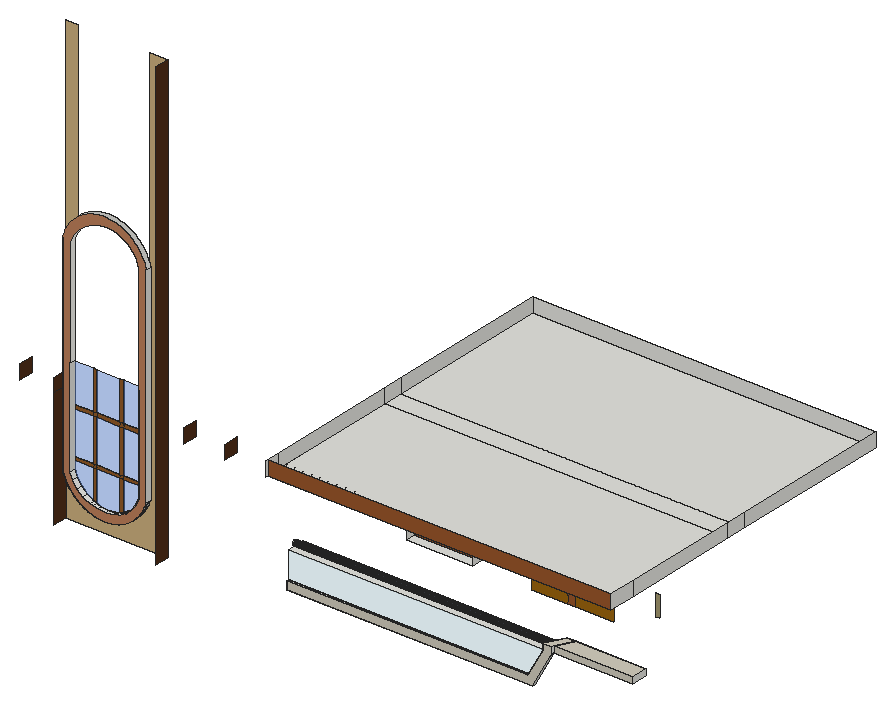
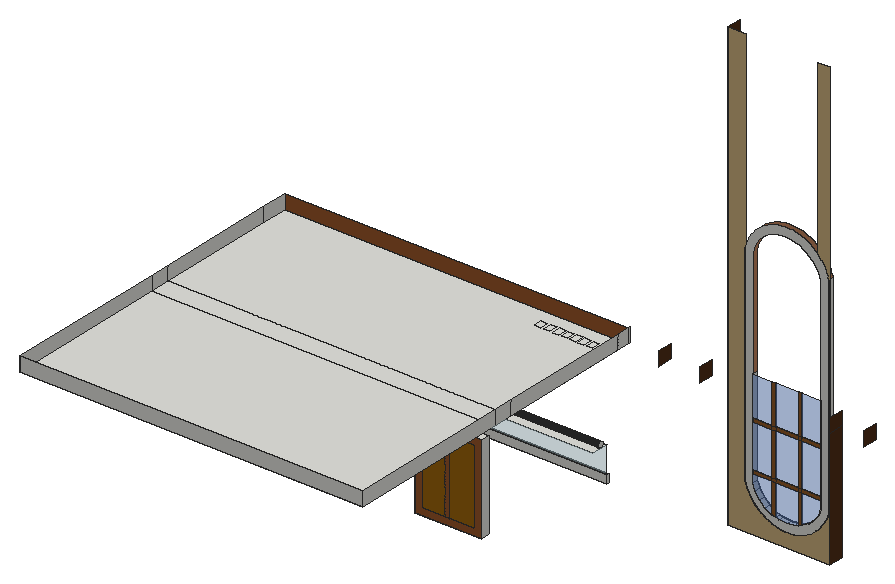
# SketchUp Ruby script. Lengths in inches.
U = 1.inch
M = Sketchup.active_model
def pt(a) = Geom::Point3d.new(a.map { |v| v * U })
def face(e, loops, mat)
  f = e.add_face(loops[0].map { |a| pt(a) })
  loops[1..].each { |l| e.add_face(l.map { |a| pt(a) }).erase! }
  f.material = f.back_material = mat if mat
  f
end
# faces: each face lists its corners as indices into pts; further lists are holes
def faces(e, pts, list, mat = nil) = list.each { |f| face(e, (f[0].is_a?(Array) ? f : [f]).map { |l| l.map { |i| pts[i] } }, mat) }
# xy, xz, yz: faces in a plane at the given z, y or x. An outline is a flat list of corners, or four numbers for a rectangle; further outlines are holes
def ring(l) = l.size == 4 ? [[l[0], l[1]], [l[2], l[1]], [l[2], l[3]], [l[0], l[3]]] : l.each_slice(2).to_a
def flat(e, list, mat, &to3) = list.each { |f| face(e, (f[0].is_a?(Array) ? f : [f]).map { |l| ring(l).map { |u, v| to3.(u, v) } }, mat) }
def xy(e, z, list, mat = nil) = flat(e, list, mat) { |x, y| [x, y, z] }
def xz(e, y, list, mat = nil) = flat(e, list, mat) { |x, z| [x, y, z] }
def yz(e, x, list, mat = nil) = flat(e, list, mat) { |y, z| [x, y, z] }
def lines(e, pts, list) = list.each { |a, b| e.add_line(pt(pts[a]), pt(pts[b])) }
# prism: a flat outline (further loops are holes) pulled along v
def prism(e, loops, v, mat = nil)
  f = face(e, loops, mat); d = Geom::Vector3d.new(v.map { |x| x * U })
  f.pushpull(f.normal.samedirection?(d) ? d.length : -d.length)
end
def box(e, o, s, mat = nil) = prism(e, [[o, [o[0] + s[0], o[1], o[2]], [o[0] + s[0], o[1] + s[1], o[2]], [o[0], o[1] + s[1], o[2]]]], [0, 0, s[2]], mat)
def at(x, y, z, deg = 0) = Geom::Transformation.translation(pt([x, y, z])) * Geom::Transformation.rotation(ORIGIN, Z_AXIS, deg.degrees)
def axes(o, x, y, z) = Geom::Transformation.new([*x, 0, *y, 0, *z, 0, *pt(o).to_a, 1])
def part(name) = M.definitions.add(name)
# library, detail: a bought-in or finely detailed component or shape, given as its bounding box
def library(name, o, s) = part(name).tap { |d| box(d.entities, o, s) }
def detail(e, o, s) = box(e.add_group.entities, o, s)
def put(e, d, t, mat = nil) = e.add_instance(d, t).tap { |i| i.material = mat if mat }
def group(e, t, mat = nil) = e.add_group.tap { |g| g.transformation = t; g.material = mat if mat }.entities
root = M.entities
M.materials.add("[Blinds Wood Light]").color = [155, 100, 14]
M.materials.add("[Formica Graystone]").color = [209, 204, 189]
M.materials.add("[Formica Laminate Dark]").color = [50, 53, 60]
M.materials.add("[Translucent Glass Blue]").color = [100, 149, 237]
M.materials["[Translucent Glass Blue]"].alpha = 0.5
M.materials.add("[Translucent Glass Safety]").color = [204, 235, 244]
M.materials["[Translucent Glass Safety]"].alpha = 0.5
M.materials.add("[Wood Board Cork]").color = [215, 201, 115]
M.materials.add("[Wood Cherry Original]").color = [152, 86, 42]
M.materials.add("[Wood Floor Light]").color = [204, 176, 127]
M.materials.add("[Wood Floor Parquet]").color = [145, 89, 39]
M.materials.add("[Wood Lumber ButtJoined]").color = [164, 152, 112]
M.materials.add("[Wood Veneer 01]").color = [79, 46, 24]
M.materials.add("[Wood Veneer 02]").color = [190, 128, 91]
xy(root,246.23,[[380.95,348.07,452.45,357.95]])
xy(root,246.97,[[356.6875,216.87,621.625,219.56]])
xy(root,255.23,[[356.6875,216.87,615.875,219.56]])
xy(root,284.4375,[[356.6875,219.56,632.125,219.56,641.9,237.64,356.6875,237.64],[632.125,219.56,641.9,237.64,651.75,237.64,641.9,219.56],[641.9,219.56,651.75,237.64,727.17,237.64,727.17,219.56]])
xy(root,291.5,[[632.125,216.87,641.9,216.87,641.9,219.56,651.75,237.64,641.9,237.64,632.125,219.56],[641.9,219.56,727.17,219.56,727.17,237.64,651.75,237.64]],"[Formica Graystone]")
xy(root,341.42,[[380.95,348.07,452.45,357.95]])
xy(root,369,[[356.6875,190.11,727.17,348.07],[358.51,205,364.9375,214.21],[367.14,205,373.5625,214.21],[376.01,205,382.4375,214.21],[385.08,205,391.5,214.21],
  [393.95,205,400.375,214.21],[403.08,205,409.5,214.21],[412.39,205,418.8125,214.21],[422.26,205,428.6875,214.21],[432.2,205,438.625,214.21],
  [356.6875,348.07,727.17,370.07],[356.6875,370.07,727.17,548.03]])
xz(root,190.11,[[356.6875,369,727.17,384.375]],"[Wood Cherry Original]")
xz(root,197.92,[[[174.5,257.11,176.5,257.16,178.5,257.29,180.5,257.5,182.48,257.8,184.45,258.18,186.4,258.65,188.33,259.2,190.24,259.83,192.11,260.54,193.96,261.33,195.76,262.2,197.53,263.15,199.26,264.17,200.94,265.26,202.58,266.43,204.16,267.66,205.6875,268.96,207.16,270.32,208.57,271.75,209.92,273.23,211.21,274.77,212.43,276.37,213.58,278.01,214.65,279.7,215.66,281.44,216.59,283.22,217.44,285.03,218.22,286.89,218.91,288.77,219.53,290.68,219.53,515.93,219.01,517.93,218.4,519.9,217.71,521.85,216.93,523.77,216.07,525.64,215.12,527.48,214.09,529.27,212.99,531.02,211.8,532.71,210.54,534.35,209.21,535.93,207.8125,537.45,206.35,538.91,204.82,540.3,203.23,541.62,201.58,542.87,199.88,544.04,198.125,545.13,196.33,546.15,194.48,547.08,192.6,547.93,190.68,548.7,188.73,549.38,186.75,549.97,184.74,550.47,182.72,550.89,180.68,551.21,178.625,551.44,176.5625,551.58,174.5,551.625,172.43,551.58,170.37,551.44,168.3125,551.21,166.27,550.89,164.25,550.47,162.24,549.97,160.26,549.38,158.3125,548.7,156.39,547.93,154.51,547.08,152.66,546.15,150.87,545.13,149.11,544.04,147.41,542.87,145.76,541.62,144.17,540.3,142.64,538.91,141.18,537.45,139.78,535.93,138.45,534.35,137.1875,532.71,136,531.02,134.9,529.27,133.87,527.48,132.92,525.64,132.06,523.77,131.28,521.85,130.59,519.9,129.98,517.93,129.46,515.93,129.46,290.68,130.08,288.77,130.77,286.89,131.55,285.03,132.4,283.22,133.33,281.44,134.34,279.7,135.41,278.01,136.5625,276.37,137.78,274.77,139.07,273.23,140.42,271.75,141.83,270.32,143.3,268.96,144.83,267.66,146.41,266.43,148.05,265.26,149.73,264.17,151.46,263.15,153.23,262.2,155.03,261.33,156.88,260.54,158.75,259.83,160.66,259.2,162.59,258.65,164.54,258.18,166.51,257.8,168.49,257.5,170.49,257.29,172.49,257.16],[174.5,265.17,166.25,266.06,161.59,267.6,158.37,268.67,151.23,272.89,145.14,278.53,140.39,285.33,137.48,292.29,137.48,514.54,141.18,522.34,146.84,529.54,153.96,535.3,156.35,536.79,161,539.58,168.71,542.1,176.79,542.85,184.83,541.79,186.27,541.26,188.66,540.38,192.4375,538.98,199.23,534.55,204.875,528.73,209.09,521.8,211.51,514.54,211.51,292.29,208.6,285.33,203.85,278.53,197.76,272.89,190.62,268.67,186.68,267.36,182.74,266.06]]],"[Wood Veneer 02]")
xz(root,203.79,[[[174.5,257.11,172.49,257.16,170.49,257.29,168.49,257.5,166.51,257.8,164.54,258.18,162.59,258.65,160.66,259.2,158.75,259.83,156.88,260.54,155.03,261.33,153.23,262.2,151.46,263.15,149.73,264.17,148.05,265.26,146.41,266.43,144.83,267.66,143.3,268.96,141.83,270.32,140.42,271.75,139.07,273.23,137.78,274.77,136.5625,276.37,135.41,278.01,134.34,279.7,133.33,281.44,132.4,283.22,131.55,285.03,130.77,286.89,130.08,288.77,129.46,290.68,129.46,515.93,129.98,517.93,130.59,519.9,131.28,521.85,132.06,523.77,132.92,525.64,133.87,527.48,134.9,529.27,136,531.02,137.1875,532.71,138.45,534.35,139.78,535.93,141.18,537.45,142.64,538.91,144.17,540.3,145.76,541.62,147.41,542.87,149.11,544.04,150.87,545.13,152.66,546.15,154.51,547.08,156.39,547.93,158.3125,548.7,160.26,549.38,162.24,549.97,164.25,550.47,166.27,550.89,168.3125,551.21,170.37,551.44,172.43,551.58,174.5,551.625,176.5625,551.58,178.625,551.44,180.68,551.21,182.72,550.89,184.74,550.47,186.75,549.97,188.73,549.38,190.68,548.7,192.6,547.93,194.48,547.08,196.33,546.15,198.125,545.13,199.88,544.04,201.58,542.87,203.23,541.62,204.82,540.3,206.35,538.91,207.8125,537.45,209.21,535.93,210.54,534.35,211.8,532.71,212.99,531.02,214.09,529.27,215.12,527.48,216.07,525.64,216.93,523.77,217.71,521.85,218.4,519.9,219.01,517.93,219.53,515.93,219.53,290.68,218.91,288.77,218.22,286.89,217.44,285.03,216.59,283.22,215.66,281.44,214.65,279.7,213.58,278.01,212.43,276.37,211.21,274.77,209.92,273.23,208.57,271.75,207.16,270.32,205.6875,268.96,204.16,267.66,202.58,266.43,200.94,265.26,199.26,264.17,197.53,263.15,195.76,262.2,193.96,261.33,192.11,260.54,190.24,259.83,188.33,259.2,186.4,258.65,184.45,258.18,182.48,257.8,180.5,257.5,178.5,257.29,176.5,257.16],[174.5,265.17,182.74,266.06,186.68,267.36,190.62,268.67,197.76,272.89,203.85,278.53,208.6,285.33,211.51,292.29,211.51,514.54,209.09,521.8,204.875,528.73,199.23,534.55,192.4375,538.98,188.66,540.38,186.27,541.26,184.83,541.79,176.79,542.85,168.71,542.1,161,539.58,156.35,536.79,153.96,535.3,146.84,529.54,141.18,522.34,137.48,514.54,137.48,292.29,140.39,285.33,145.14,278.53,151.23,272.89,158.37,268.67,161.59,267.6,166.25,266.06]]])
xz(root,203.79,[[174.5,265.17,182.74,266.06,186.68,267.36,186.68,300.8,161.59,300.8,161.59,267.6,166.25,266.06],[158.37,268.67,158.37,300.8,137.48,300.8,137.48,292.29,140.39,285.33,145.14,278.53,151.23,272.89],[190.62,268.67,197.76,272.89,203.85,278.53,208.6,285.33,211.51,292.29,211.51,300.8,190.62,300.8],[137.48,304.36,158.37,350.71],[161.59,304.36,186.68,350.71],
  [190.62,304.36,211.51,350.71],[137.48,354.75,158.37,397.07],[161.59,354.75,186.68,397.07],[190.62,354.75,211.51,397.07]],"[Translucent Glass Blue]")
xz(root,203.79,[[128,242.08,238.01,242.08,238.01,723.1875,218.4,723.1875,218.4,519.9,219.01,517.93,219.53,515.93,219.53,290.68,218.91,288.77,218.22,286.89,217.44,285.03,216.59,283.22,215.66,281.44,214.65,279.7,213.58,278.01,212.43,276.37,211.21,274.77,209.92,273.23,208.57,271.75,207.16,270.32,205.6875,268.96,204.16,267.66,202.58,266.43,200.94,265.26,199.26,264.17,197.53,263.15,195.76,262.2,193.96,261.33,192.11,260.54,190.24,259.83,188.33,259.2,186.4,258.65,184.45,258.18,182.48,257.8,180.5,257.5,178.5,257.29,176.5,257.16,174.5,257.11,172.49,257.16,170.49,257.29,168.49,257.5,166.51,257.8,164.54,258.18,162.59,258.65,160.66,259.2,158.75,259.83,156.88,260.54,155.03,261.33,153.23,262.2,151.46,263.15,149.73,264.17,148.05,265.26,146.41,266.43,144.83,267.66,143.3,268.96,141.83,270.32,140.42,271.75,139.07,273.23,137.78,274.77,136.5625,276.37,135.41,278.01,134.34,279.7,133.33,281.44,132.4,283.22,131.55,285.03,130.77,286.89,130.08,288.77,129.46,290.68,129.46,515.93,129.98,517.93,130.59,519.9,131.28,521.85,132.06,523.77,132.92,525.64,133.87,527.48,134.9,529.27,136,531.02,137.1875,532.71,138.45,534.35,139.78,535.93,141.18,537.45,141.18,723.1875,128,723.1875]],"[Wood Floor Light]")
xz(root,203.79,[[186.68,267.36,190.62,268.67,190.62,300.8,186.68,300.8],[161.59,267.6,161.59,300.8,158.37,300.8,158.37,268.67],[137.48,300.8,158.37,304.36],[158.37,300.8,161.59,304.36],[161.59,300.8,186.68,304.36],
  [186.68,300.8,190.62,304.36],[190.62,300.8,211.51,304.36],[158.37,304.36,161.59,350.71],[186.68,304.36,190.62,350.71],[137.48,350.71,158.37,354.75],
  [158.37,350.71,161.59,354.75],[161.59,350.71,186.68,354.75],[186.68,350.71,190.62,354.75],[190.62,350.71,211.51,354.75],[158.37,354.75,161.59,397.07],
  [186.68,354.75,190.62,397.07]],"[Wood Floor Parquet]")
xz(root,216.87,[[356.6875,246.97,621.625,246.97,640.93,282.64,641.9,284.4375,641.9,291.5,632.125,291.5,632.125,284.4375,615.875,255.23,356.6875,255.23]],"[Formica Graystone]")
xz(root,219.56,[[356.6875,246.97,356.6875,255.23,615.875,255.23,632.125,284.4375,641.9,284.4375,640.93,282.64,621.625,246.97]])
xz(root,219.56,[[641.9,284.4375,727.17,291.5]],"[Formica Graystone]")
xz(root,219.56,[[356.6875,255.23,615.875,255.23,632.125,284.4375,356.6875,284.4375]],"[Translucent Glass Safety]")
xz(root,237.64,[[641.9,284.4375,651.75,291.5],[651.75,284.4375,727.17,291.5]])
xz(root,348.07,[[515.72,244.91,555.02,333.92],[563.01,244.91,604.72,333.92]],"[Blinds Wood Light]")
xz(root,348.07,[[642.89,296.77,696.74,345.62,691.75,345.62,672.61,328.45,669.91,326.02,642.89,301.77],[669.91,326.02,672.61,328.45,652.63,345.62,648.8,345.62]],"[Wood Board Cork]")
xz(root,348.07,[[555.02,244.91,563.01,333.92]],"[Wood Cherry Original]")
xz(root,348.07,[[642.89,301.77,669.91,326.02,648.8,345.62,642.89,345.62],[672.61,328.45,691.75,345.62,652.63,345.62]],"[Wood Floor Light]")
xz(root,348.07,[[649.28,265.99,653.91,288.67]],"[Wood Lumber ButtJoined]")
xz(root,357.95,[[387.91,253.1875,414.49,334.46],[420.72,253.1875,445.5,334.46]],"[Blinds Wood Light]")
xz(root,357.95,[[[380.95,246.23,452.45,341.42],[387.91,253.1875,445.5,334.46]],[414.49,253.1875,420.72,334.46]],"[Wood Cherry Original]")
xz(root,548.03,[[356.6875,369,727.17,384.375]])
yz(root,91,[[188.11,369,203.79,384.375]],"[Wood Veneer 01]")
yz(root,128,[[188.11,242.08,203.79,369],[188.11,369,203.79,384.375]],"[Wood Veneer 01]")
yz(root,129.46,[[197.92,290.68,203.79,515.93]])
yz(root,137.48,[[197.92,292.29,203.79,397.07]])
yz(root,211.51,[[197.92,292.29,203.79,397.07]])
yz(root,219.53,[[197.92,290.68,203.79,515.93]])
yz(root,238.01,[[188.11,242.08,203.79,723.1875]],"[Wood Veneer 01]")
yz(root,267.9375,[[188.11,369,203.79,384.375]],"[Wood Veneer 01]")
yz(root,312.3125,[[188.11,369,203.79,384.375]],"[Wood Veneer 01]")
yz(root,356.6875,[[216.87,246.97,219.56,255.23],[227.13,285.1,226.4,285.19,225.72,285.47,225.14,285.92,224.69,286.5,224.41,287.18,224.32,287.91,224.41,288.64,224.69,289.32,225.14,289.9,225.72,290.35,226.4,290.625,227.13,290.72,227.86,290.625,228.54,290.35,229.12,289.9,229.57,289.32,229.85,288.64,229.94,287.91,229.85,287.18,229.57,286.5,229.12,285.92,228.54,285.47,227.86,285.19],[188.11,369,190.11,384.375],[190.11,369,203.79,384.375],[203.79,369,348.07,384.375],
  [348.07,369,370.07,384.375],[370.07,369,548.03,384.375]])
yz(root,380.95,[[348.07,246.23,357.95,341.42]])
yz(root,452.45,[[348.07,246.23,357.95,341.42]])
yz(root,632.125,[[216.87,284.4375,219.56,291.5]])
yz(root,636.17,[[227.13,285.1,227.86,285.19,228.54,285.47,229.12,285.92,229.57,286.5,229.85,287.18,229.94,287.91,229.85,288.64,229.57,289.32,229.12,289.9,228.54,290.35,227.86,290.625,227.13,290.72,226.4,290.625,225.72,290.35,225.14,289.9,224.69,289.32,224.41,288.64,224.32,287.91,224.41,287.18,224.69,286.5,225.14,285.92,225.72,285.47,226.4,285.19]])
yz(root,641.9,[[216.87,284.4375,219.56,291.5]])
yz(root,727.17,[[219.56,284.4375,237.64,291.5],[190.11,369,219.56,384.375],[219.56,369,348.07,384.375],[348.07,369,370.07,384.375],[370.07,369,548.03,384.375]])
p = [[621.625,219.56,246.97],[640.93,219.56,282.64],[640.93,216.87,282.64],[621.625,216.87,246.97],[632.125,219.56,284.4375],[615.875,219.56,255.23],
  [615.875,216.87,255.23],[632.125,216.87,284.4375],[172.49,203.79,257.16],[174.5,203.79,257.11],[174.5,197.92,257.11],[172.49,197.92,257.16],
  [176.5,203.79,257.16],[176.5,197.92,257.16],[170.49,203.79,257.29],[170.49,197.92,257.29],[178.5,203.79,257.29],[178.5,197.92,257.29],
  [168.49,203.79,257.5],[168.49,197.92,257.5],[180.5,203.79,257.5],[180.5,197.92,257.5],[166.51,203.79,257.8],[166.51,197.92,257.8],
  [182.48,203.79,257.8],[182.48,197.92,257.8],[164.54,203.79,258.18],[164.54,197.92,258.18],[184.45,203.79,258.18],[184.45,197.92,258.18],
  [162.59,203.79,258.65],[162.59,197.92,258.65],[186.4,203.79,258.65],[186.4,197.92,258.65],[160.66,203.79,259.2],[160.66,197.92,259.2],
  [188.33,203.79,259.2],[188.33,197.92,259.2],[158.75,203.79,259.83],[158.75,197.92,259.83],[190.24,203.79,259.83],[190.24,197.92,259.83],
  [156.88,203.79,260.54],[156.88,197.92,260.54],[192.11,203.79,260.54],[192.11,197.92,260.54],[155.03,203.79,261.33],[155.03,197.92,261.33],
  [193.96,203.79,261.33],[193.96,197.92,261.33],[153.23,203.79,262.2],[153.23,197.92,262.2],[195.76,203.79,262.2],[195.76,197.92,262.2],
  [151.46,203.79,263.15],[151.46,197.92,263.15],[197.53,203.79,263.15],[197.53,197.92,263.15],[149.73,203.79,264.17],[149.73,197.92,264.17],
  [199.26,203.79,264.17],[199.26,197.92,264.17],[148.05,203.79,265.26],[148.05,197.92,265.26],[200.94,203.79,265.26],[200.94,197.92,265.26],
  [174.5,203.79,265.17],[166.25,203.79,266.06],[166.25,197.92,266.06],[174.5,197.92,265.17],[182.74,203.79,266.06],[182.74,197.92,266.06],
  [146.41,203.79,266.43],[146.41,197.92,266.43],[202.58,203.79,266.43],[202.58,197.92,266.43],[161.59,203.79,267.6],[161.59,197.92,267.6],
  [186.68,203.79,267.36],[186.68,197.92,267.36],[144.83,203.79,267.66],[144.83,197.92,267.66],[204.16,203.79,267.66],[204.16,197.92,267.66],
  [190.62,203.79,268.67],[190.62,197.92,268.67],[158.37,203.79,268.67],[158.37,197.92,268.67],[143.3,203.79,268.96],[143.3,197.92,268.96],
  [205.6875,203.79,268.96],[205.6875,197.92,268.96],[151.23,203.79,272.89],[151.23,197.92,272.89],[197.76,203.79,272.89],[197.76,197.92,272.89],
  [141.83,203.79,270.32],[141.83,197.92,270.32],[207.16,203.79,270.32],[207.16,197.92,270.32],[140.42,203.79,271.75],[140.42,197.92,271.75],
  [208.57,203.79,271.75],[208.57,197.92,271.75],[139.07,203.79,273.23],[139.07,197.92,273.23],[209.92,203.79,273.23],[209.92,197.92,273.23],
  [145.14,203.79,278.53],[145.14,197.92,278.53],[203.85,203.79,278.53],[203.85,197.92,278.53],[137.78,203.79,274.77],[137.78,197.92,274.77],
  [211.21,203.79,274.77],[211.21,197.92,274.77],[136.5625,203.79,276.37],[136.5625,197.92,276.37],[212.43,203.79,276.37],[212.43,197.92,276.37],
  [135.41,203.79,278.01],[135.41,197.92,278.01],[213.58,203.79,278.01],[213.58,197.92,278.01],[134.34,203.79,279.7],[134.34,197.92,279.7],
  [214.65,203.79,279.7],[214.65,197.92,279.7],[140.39,203.79,285.33],[140.39,197.92,285.33],[208.6,203.79,285.33],[208.6,197.92,285.33],
  [133.33,203.79,281.44],[133.33,197.92,281.44],[215.66,203.79,281.44],[215.66,197.92,281.44],[132.4,203.79,283.22],[132.4,197.92,283.22],
  [216.59,203.79,283.22],[216.59,197.92,283.22],[641.9,219.56,284.4375],[641.9,216.87,284.4375],[131.55,203.79,285.03],[131.55,197.92,285.03],
  [217.44,203.79,285.03],[217.44,197.92,285.03],[641.9,237.64,284.4375],[632.125,219.56,291.5],[641.9,237.64,291.5],[651.75,237.64,284.4375],
  [641.9,219.56,291.5],[651.75,237.64,291.5],[130.77,203.79,286.89],[130.77,197.92,286.89],[218.22,203.79,286.89],[218.22,197.92,286.89],
  [356.6875,226.4,285.19],[356.6875,227.13,285.1],[636.17,227.13,285.1],[636.17,226.4,285.19],[356.6875,227.86,285.19],[636.17,227.86,285.19],
  [356.6875,225.72,285.47],[636.17,225.72,285.47],[356.6875,228.54,285.47],[636.17,228.54,285.47],[137.48,203.79,292.29],[137.48,197.92,292.29],
  [211.51,203.79,292.29],[211.51,197.92,292.29],[356.6875,225.14,285.92],[636.17,225.14,285.92],[356.6875,229.12,285.92],[636.17,229.12,285.92],
  [356.6875,224.69,286.5],[636.17,224.69,286.5],[356.6875,229.57,286.5],[636.17,229.57,286.5],[356.6875,224.41,287.18],[636.17,224.41,287.18],
  [356.6875,229.85,287.18],[636.17,229.85,287.18],[130.08,203.79,288.77],[130.08,197.92,288.77],[218.91,203.79,288.77],[218.91,197.92,288.77],
  [356.6875,224.32,287.91],[636.17,224.32,287.91],[356.6875,229.94,287.91],[636.17,229.94,287.91],[356.6875,224.41,288.64],[636.17,224.41,288.64],
  [356.6875,229.85,288.64],[636.17,229.85,288.64],[356.6875,224.69,289.32],[636.17,224.69,289.32],[356.6875,229.57,289.32],[636.17,229.57,289.32],
  [129.46,203.79,290.68],[129.46,197.92,290.68],[219.53,203.79,290.68],[219.53,197.92,290.68],[356.6875,225.14,289.9],[636.17,225.14,289.9],
  [356.6875,229.12,289.9],[636.17,229.12,289.9],[356.6875,225.72,290.35],[636.17,225.72,290.35],[356.6875,228.54,290.35],[636.17,228.54,290.35],
  [356.6875,226.4,290.625],[636.17,226.4,290.625],[356.6875,227.86,290.625],[636.17,227.86,290.625],[356.6875,227.13,290.72],[636.17,227.13,290.72]]
faces(root,p,[[0,1,2,3],[4,5,6,7],[8,9,10,11],[9,12,13,10],[14,8,11,15],[12,16,17,13],[18,14,15,19],[16,20,21,17],
  [22,18,19,23],[20,24,25,21],[26,22,23,27],[24,28,29,25],[30,26,27,31],[28,32,33,29],[34,30,31,35],[32,36,37,33],
  [38,34,35,39],[36,40,41,37],[42,38,39,43],[40,44,45,41],[46,42,43,47],[44,48,49,45],[50,46,47,51],[48,52,53,49],
  [54,50,51,55],[52,56,57,53],[58,54,55,59],[56,60,61,57],[62,58,59,63],[60,64,65,61],[66,67,68,69],[70,66,69,71],
  [72,62,63,73],[64,74,75,65],[67,76,77,68],[78,70,71,79],[80,72,73,81],[74,82,83,75],[84,78,79,85],[76,86,87,77],
  [88,80,81,89],[82,90,91,83],[86,92,93,87],[94,84,85,95],[96,88,89,97],[90,98,99,91],[100,96,97,101],[98,102,103,99],
  [104,100,101,105],[102,106,107,103],[92,108,109,93],[110,94,95,111],[112,104,105,113],[106,114,115,107],[116,112,113,117],[114,118,119,115],
  [120,116,117,121],[118,122,123,119],[124,120,121,125],[122,126,127,123],[108,128,129,109],[130,110,111,131],[132,124,125,133],[126,134,135,127],
  [136,132,133,137],[134,138,139,135],[1,140,141,2],[142,136,137,143],[138,144,145,139],[146,4,147,148],[149,140,150,151],[152,142,143,153],
  [144,154,155,145],[128,166,167,129],[168,130,131,169],[182,152,153,183],[154,184,185,155],[198,182,183,199],[184,200,201,185]])
faces(root,p,[[156,157,158,159],[157,160,161,158],[162,156,159,163],[160,164,165,161],[170,162,163,171],[164,172,173,165],[174,170,171,175],[172,176,177,173],
  [178,174,175,179],[176,180,181,177],[186,178,179,187],[180,188,189,181],[190,186,187,191],[188,192,193,189],[194,190,191,195],[192,196,197,193],
  [202,194,195,203],[196,204,205,197],[206,202,203,207],[204,208,209,205],[210,206,207,211],[208,212,213,209],[214,210,211,215],[212,214,215,213]],"[Formica Laminate Dark]")
